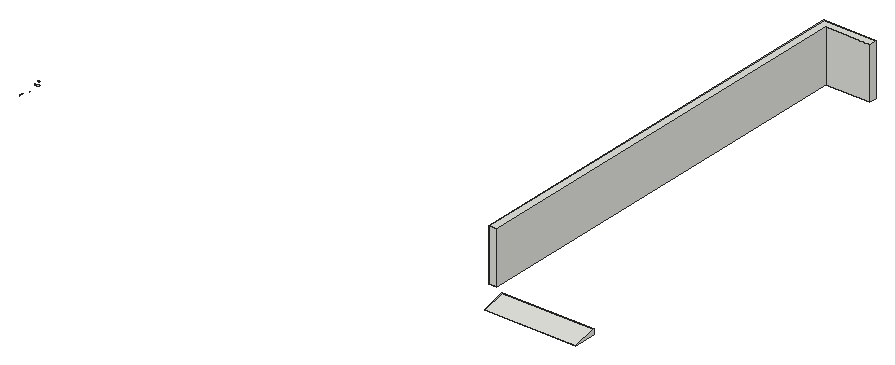
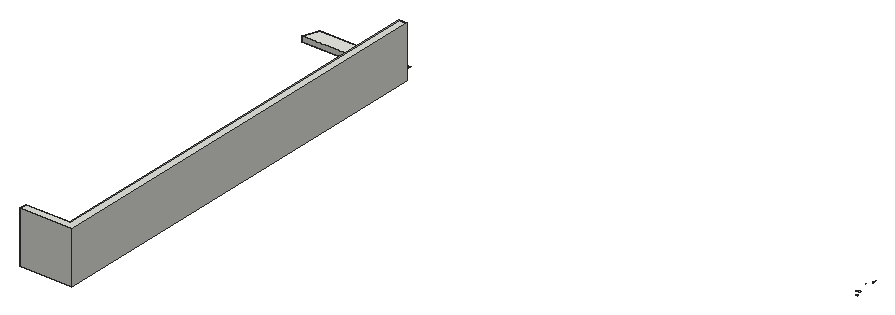
# SketchUp Ruby script. Lengths in inches.
U = 1.inch
M = Sketchup.active_model
def pt(a) = Geom::Point3d.new(a.map { |v| v * U })
def face(e, loops, mat)
  f = e.add_face(loops[0].map { |a| pt(a) })
  loops[1..].each { |l| e.add_face(l.map { |a| pt(a) }).erase! }
  f.material = f.back_material = mat if mat
  f
end
# faces: each face lists its corners as indices into pts; further lists are holes
def faces(e, pts, list, mat = nil) = list.each { |f| face(e, (f[0].is_a?(Array) ? f : [f]).map { |l| l.map { |i| pts[i] } }, mat) }
# xy, xz, yz: faces in a plane at the given z, y or x. An outline is a flat list of corners, or four numbers for a rectangle; further outlines are holes
def ring(l) = l.size == 4 ? [[l[0], l[1]], [l[2], l[1]], [l[2], l[3]], [l[0], l[3]]] : l.each_slice(2).to_a
def flat(e, list, mat, &to3) = list.each { |f| face(e, (f[0].is_a?(Array) ? f : [f]).map { |l| ring(l).map { |u, v| to3.(u, v) } }, mat) }
def xy(e, z, list, mat = nil) = flat(e, list, mat) { |x, y| [x, y, z] }
def xz(e, y, list, mat = nil) = flat(e, list, mat) { |x, z| [x, y, z] }
def yz(e, x, list, mat = nil) = flat(e, list, mat) { |y, z| [x, y, z] }
def lines(e, pts, list) = list.each { |a, b| e.add_line(pt(pts[a]), pt(pts[b])) }
# prism: a flat outline (further loops are holes) pulled along v
def prism(e, loops, v, mat = nil)
  f = face(e, loops, mat); d = Geom::Vector3d.new(v.map { |x| x * U })
  f.pushpull(f.normal.samedirection?(d) ? d.length : -d.length)
end
def box(e, o, s, mat = nil) = prism(e, [[o, [o[0] + s[0], o[1], o[2]], [o[0] + s[0], o[1] + s[1], o[2]], [o[0], o[1] + s[1], o[2]]]], [0, 0, s[2]], mat)
def at(x, y, z, deg = 0) = Geom::Transformation.translation(pt([x, y, z])) * Geom::Transformation.rotation(ORIGIN, Z_AXIS, deg.degrees)
def axes(o, x, y, z) = Geom::Transformation.new([*x, 0, *y, 0, *z, 0, *pt(o).to_a, 1])
def part(name) = M.definitions.add(name)
# library, detail: a bought-in or finely detailed component or shape, given as its bounding box
def library(name, o, s) = part(name).tap { |d| box(d.entities, o, s) }
def detail(e, o, s) = box(e.add_group.entities, o, s)
def put(e, d, t, mat = nil) = e.add_instance(d, t).tap { |i| i.material = mat if mat }
def group(e, t, mat = nil) = e.add_group.tap { |g| g.transformation = t; g.material = mat if mat }.entities
root = M.entities
prism(root,[[[600.961,339.2731,0],[600.961,313.8509,0],[600.961,339.2731,6]]],[105.6875,0,0])
xy(root,0,[[26.9831,360.1386,26.9873,360.1387,26.9915,360.1392,26.9957,360.14,26.9998,360.141,27.0039,360.1424,27.0078,360.144,27.0095,360.1449,27.0112,360.1459,27.0128,360.147,27.0143,360.1482,27.0158,360.1495,27.0172,360.1509,27.0196,360.1539,27.0207,360.1556,27.0225,360.159,27.0234,360.1614,27.0242,360.1639,27.0248,360.1663,27.0252,360.1689,27.0255,360.1714,27.0256,360.174,27.0254,360.1765,27.0251,360.1791,27.0247,360.1816,27.0232,360.1872,27.0214,360.1927,27.0192,360.198,27.0166,360.2032,27.0138,360.2082,26.995,360.2348,26.9851,360.2465,26.9744,360.2573,26.9648,360.2657,26.9547,360.2732,26.9533,360.2742,26.9517,360.275,26.9502,360.2757,26.9486,360.2764,26.9469,360.2769,26.9452,360.2773,26.9435,360.2776,26.9401,360.2778,26.939,360.2778,26.9379,360.2776,26.9368,360.2775,26.9357,360.2772,26.9347,360.2768,26.9336,360.2764,26.9326,360.276,26.9308,360.2748,26.9299,360.2741,26.9291,360.2734,26.9283,360.2726,26.9254,360.2691,26.9227,360.2654,26.9204,360.2615,26.9184,360.2573,26.9155,360.25,26.9132,360.2425,26.9116,360.2348,26.9099,360.2216,26.9094,360.2082,26.9095,360.2036,26.91,360.1991,26.9108,360.1946,26.9119,360.1902,26.9133,360.1859,26.915,360.1816,26.917,360.1775,26.9193,360.1734,26.9219,360.1695,26.9247,360.1658,26.9277,360.1623,26.931,360.159,26.9353,360.1553,26.9399,360.1519,26.9447,360.1488,26.9497,360.1462,26.9549,360.1439,26.9604,360.142,26.9659,360.1405,26.9716,360.1394,26.9773,360.1388],[27.1858,360.1773,27.1887,360.1773,27.1901,360.1774,27.1929,360.178,27.1943,360.1784,27.1956,360.1789,27.1969,360.1795,27.1998,360.1811,27.2026,360.1829,27.2053,360.1848,27.2078,360.187,27.2101,360.1893,27.2123,360.1918,27.2143,360.1944,27.2161,360.1972,27.2209,360.2058,27.225,360.2147,27.2284,360.2239,27.231,360.2334,27.2357,360.2578,27.2386,360.2826,27.243,360.3857,27.2429,360.3876,27.2427,360.3896,27.2424,360.3915,27.242,360.3934,27.2414,360.3952,27.2407,360.397,27.2398,360.3988,27.2389,360.4005,27.2367,360.4037,27.2354,360.4051,27.234,360.4065,27.2326,360.4078,27.231,360.409,27.2294,360.41,27.2277,360.411,27.2259,360.4118,27.2247,360.4123,27.2223,360.4129,27.221,360.4132,27.2198,360.4133,27.2172,360.4133,27.216,360.4132,27.2147,360.413,27.2135,360.4127,27.2111,360.4119,27.2099,360.4114,27.2088,360.4108,27.2077,360.4101,27.2057,360.4085,27.2039,360.4067,27.2031,360.4057,27.2024,360.4047,27.2017,360.4036,27.2012,360.4025,27.1634,360.3148,27.1588,360.3013,27.1551,360.2874,27.1523,360.2734,27.1508,360.26,27.1503,360.2466,27.1511,360.2332,27.1522,360.2248,27.154,360.2165,27.1563,360.2083,27.1593,360.2004,27.1606,360.1977,27.162,360.1951,27.1636,360.1926,27.1653,360.1902,27.1673,360.188,27.1693,360.1859,27.1716,360.1839,27.1739,360.1821,27.1764,360.1804,27.1776,360.1797,27.1789,360.1791,27.1802,360.1786,27.1816,360.1781,27.1844,360.1775],[27.1335,363.4794,27.1354,363.4795,27.1373,363.4797,27.1392,363.48,27.1411,363.4804,27.1429,363.481,27.1447,363.4817,27.1464,363.4825,27.1481,363.4834,27.1513,363.4856,27.1541,363.4882,27.1563,363.4908,27.1572,363.4923,27.1581,363.4937,27.1588,363.4953,27.16,363.4985,27.1604,363.5001,27.1608,363.5035,27.1609,363.5052,27.1608,363.5069,27.1606,363.5086,27.1595,363.5144,27.1581,363.5202,27.1563,363.5258,27.154,363.5312,27.1514,363.5366,27.1485,363.5417,27.134,363.5633,27.1182,363.5838,27.0868,363.6242,27.0646,363.6591,27.0582,363.6718,27.0525,363.6858,27.0523,363.6871,27.0524,363.6884,27.0528,363.6896,27.0533,363.6907,27.0541,363.6917,27.0551,363.6925,27.0562,363.6931,27.0574,363.6935,27.2123,363.7212,27.2434,363.7248,27.2746,363.726,27.3059,363.725,27.3164,363.7239,27.3268,363.7221,27.3371,363.7196,27.3471,363.7163,27.357,363.7124,27.3665,363.7079,27.3728,363.7043,27.3789,363.7004,27.3846,363.696,27.3901,363.6913,27.3953,363.6862,27.4,363.6807,27.4044,363.675,27.4085,363.669,27.4134,363.6615,27.4188,363.6544,27.4247,363.6477,27.431,363.6413,27.4349,363.6379,27.439,363.6347,27.4433,363.6319,27.4478,363.6293,27.4525,363.627,27.4572,363.625,27.4608,363.6239,27.4644,363.623,27.468,363.6223,27.4717,363.622,27.4754,363.6219,27.4791,363.622,27.4828,363.6225,27.4855,363.623,27.4881,363.6237,27.4906,363.6246,27.4931,363.6257,27.4955,363.6269,27.4979,363.6283,27.5001,363.6298,27.5022,363.6315,27.5041,363.6334,27.5072,363.6367,27.51,363.6401,27.5125,363.6438,27.5148,363.6477,27.5167,363.6517,27.5184,363.6559,27.5207,363.6631,27.5224,363.6704,27.5235,363.6779,27.524,363.6854,27.524,363.6935,27.5234,363.7015,27.5222,363.7095,27.5204,363.7173,27.5181,363.725,27.5152,363.7325,27.5118,363.7397,27.5078,363.7466,27.5013,363.7564,27.4942,363.7657,27.4864,363.7744,27.478,363.7826,27.469,363.7902,27.4596,363.7971,27.4497,363.8034,27.4393,363.809,27.4286,363.8138,27.149,363.9215,26.881,364.0111,26.8784,364.0117,26.877,364.0119,26.8757,364.012,26.8743,364.012,26.873,364.0119,26.8716,364.0117,26.869,364.0111,26.8677,364.0107,26.8664,364.0101,26.864,364.0089,26.8618,364.0073,26.8608,364.0064,26.8598,364.0054,26.8589,364.0044,26.8573,364.0022,26.8561,363.9998,26.8556,363.9985,26.8551,363.9973,26.8548,363.9959,26.8545,363.9946,26.8543,363.9933,26.8543,363.9892,26.8545,363.9879,26.8548,363.9865,26.8556,363.9839,26.8561,363.9827,26.8567,363.9815,26.8719,363.9503,26.9019,363.8799,26.9367,363.7958,26.9729,363.7056,27.0123,363.619,27.0333,363.5816,27.0569,363.5458,27.0776,363.5189,27.1003,363.4935,27.1025,363.4913,27.1049,363.4893,27.1074,363.4875,27.11,363.4859,27.1127,363.4844,27.1155,363.4831,27.1183,363.482,27.1213,363.481,27.1243,363.4803,27.1273,363.4798,27.1304,363.4795],[27.6414,363.8505,27.6432,363.8505,27.6451,363.8506,27.6469,363.8509,27.6487,363.8513,27.6504,363.8518,27.6522,363.8525,27.6538,363.8532,27.6555,363.8541,27.6574,363.8553,27.6592,363.8566,27.6609,363.8581,27.6625,363.8596,27.664,363.8613,27.6654,363.863,27.6678,363.8668,27.6688,363.8688,27.6696,363.8709,27.6703,363.873,27.6709,363.8752,27.6713,363.8774,27.6716,363.8796,27.675,363.9581,27.6741,363.9777,27.6716,363.9971,27.6674,364.0163,27.6644,364.0263,27.6606,364.0362,27.6562,364.0457,27.651,364.055,27.6453,364.0638,27.6406,364.0699,27.6355,364.0757,27.6301,364.081,27.6242,364.086,27.618,364.0906,27.6115,364.0947,27.6068,364.0973,27.6019,364.0995,27.5969,364.1014,27.5918,364.103,27.5866,364.1042,27.5813,364.1051,27.5759,364.1056,27.5706,364.1058,27.5571,364.1053,27.5438,364.1038,27.5306,364.1013,27.5218,364.0989,27.5132,364.0958,27.5049,364.0922,27.4968,364.0879,27.4917,364.0846,27.4869,364.081,27.4823,364.077,27.4781,364.0726,27.4742,364.068,27.4727,364.066,27.4714,364.0639,27.4702,364.0617,27.4691,364.0594,27.4682,364.057,27.4675,364.0546,27.4669,364.0522,27.4665,364.0497,27.4662,364.0472,27.4662,364.0447,27.4663,364.0404,27.4667,364.036,27.4675,364.0317,27.4685,364.0275,27.4698,364.0234,27.4713,364.0193,27.4732,364.0154,27.4843,363.9953,27.4968,363.9761,27.513,363.9548,27.5306,363.9347,27.5706,363.897,27.6275,363.8548,27.6307,363.853,27.6324,363.8523,27.6341,363.8517,27.6359,363.8512,27.6377,363.8508,27.6395,363.8506],[29.9973,370.1849,29.9984,370.185,29.9995,370.1853,30.0005,370.1857,30.0015,370.1862,30.0024,370.1869,30.0032,370.1877,30.0039,370.1885,30.0097,370.1978,30.0149,370.2075,30.0193,370.2175,30.0238,370.23,30.0274,370.2427,30.0302,370.2556,30.032,370.2685,30.0328,370.2814,30.0328,370.2944,30.0318,370.3058,30.03,370.3171,30.0273,370.3282,30.0261,370.3318,30.0246,370.3353,30.0229,370.3388,30.021,370.342,30.0188,370.3452,30.0164,370.3481,30.0131,370.3516,30.0116,370.3528,30.0099,370.3537,30.0081,370.3544,30.0062,370.3549,30.0043,370.3551,30.0023,370.3551,30.0004,370.3547,29.9986,370.3542,29.9972,370.3536,29.9958,370.3528,29.9944,370.3521,29.9932,370.3512,29.992,370.3502,29.9908,370.3491,29.9898,370.348,29.9888,370.3468,29.9879,370.3456,29.9871,370.3442,29.9864,370.3429,29.9857,370.3415,29.9828,370.3333,29.9806,370.325,29.979,370.3166,29.978,370.308,29.9773,370.2596,29.9814,370.2076,29.9817,370.2054,29.9822,370.2031,29.9828,370.2009,29.9836,370.1988,29.9856,370.1946,29.9868,370.1927,29.9882,370.1908,29.9896,370.189,29.9912,370.1873,29.992,370.1866,29.993,370.186,29.994,370.1855,29.995,370.1852,29.9961,370.185],
  [26.9652,383.6659,26.9695,383.6661,26.9738,383.6665,26.978,383.6673,26.9822,383.6683,26.9848,383.6692,26.9874,383.6702,26.9899,383.6714,26.9923,383.6728,26.9946,383.6743,26.9968,383.676,26.9989,383.6779,27.0008,383.6798,27.0026,383.6819,27.0043,383.6841,27.0058,383.6865,27.0072,383.6889,27.0083,383.6914,27.0093,383.694,27.0102,383.6966,27.0108,383.6993,27.0113,383.702,27.0115,383.7048,27.0116,383.7076,27.0101,383.7396,27.0059,383.7713,26.9991,383.8026,26.9957,383.8178,26.9933,383.8332,26.9919,383.8488,26.9915,383.8644,26.9922,383.88,26.9939,383.8955,26.9945,383.8987,26.9952,383.9019,26.9962,383.905,26.9974,383.9081,26.9988,383.911,27.0004,383.9139,27.0022,383.9166,27.0042,383.9192,27.0063,383.9217,27.0086,383.924,27.011,383.9262,27.0136,383.9282,27.0163,383.93,27.0191,383.9317,27.022,383.9331,27.025,383.9344,27.0281,383.9354,27.0313,383.9363,27.0345,383.9369,27.0418,383.9378,27.0492,383.9383,27.0565,383.9382,27.0639,383.9376,27.0712,383.9366,27.0784,383.935,27.0855,383.9329,27.0924,383.9304,27.0991,383.9274,27.1057,383.924,27.1119,383.9201,27.1643,383.8812,27.2126,383.8374,27.2555,383.7974,27.298,383.7637,27.3353,383.739,27.3378,383.7376,27.3403,383.7364,27.343,383.7354,27.3457,383.7345,27.3484,383.7339,27.3512,383.7334,27.354,383.7331,27.3568,383.733,27.358,383.733,27.3593,383.7332,27.3605,383.7334,27.3618,383.7337,27.363,383.734,27.3641,383.7345,27.3653,383.735,27.3675,383.7362,27.3695,383.7378,27.3704,383.7386,27.3712,383.7396,27.372,383.7405,27.3759,383.746,27.3793,383.7516,27.3823,383.7576,27.3849,383.7637,27.3886,383.7747,27.3916,383.786,27.3937,383.7974,27.3958,383.8173,27.3966,383.8374,27.3971,383.8508,27.3989,383.8642,27.4018,383.8773,27.4039,383.8844,27.4065,383.8914,27.4096,383.8982,27.4131,383.9048,27.417,383.9111,27.4201,383.9155,27.4235,383.9196,27.4272,383.9236,27.4311,383.9272,27.4353,383.9306,27.4396,383.9337,27.4426,383.9356,27.4457,383.9372,27.449,383.9386,27.4523,383.9397,27.4557,383.9406,27.4592,383.9413,27.4626,383.9417,27.4662,383.9418,27.4697,383.9417,27.4732,383.9413,27.4766,383.9406,27.48,383.9397,27.4834,383.9386,27.4866,383.9372,27.4897,383.9356,27.4927,383.9337,27.4971,383.9306,27.5012,383.9272,27.5051,383.9236,27.5088,383.9196,27.5122,383.9155,27.5153,383.9111,27.5192,383.9048,27.5227,383.8982,27.5258,383.8914,27.5284,383.8844,27.5306,383.8773,27.5334,383.8642,27.5352,383.8508,27.5358,383.8374,27.5361,383.8275,27.5372,383.8176,27.5389,383.8078,27.5414,383.7982,27.5445,383.7888,27.5483,383.7796,27.5527,383.7707,27.5552,383.7666,27.558,383.7626,27.561,383.7588,27.5643,383.7552,27.5678,383.7518,27.5715,383.7487,27.5755,383.7459,27.5796,383.7434,27.584,383.7411,27.5884,383.7392,27.593,383.7376,27.5977,383.7363,27.6026,383.7353,27.6075,383.7346,27.6125,383.7342,27.6175,383.7342,27.6225,383.7345,27.6275,383.7352,27.6324,383.7361,27.6372,383.7374,27.6419,383.739,27.6466,383.7409,27.6511,383.7431,27.6554,383.7456,27.664,383.7514,27.6721,383.7577,27.6799,383.7645,27.6872,383.7718,27.694,383.7796,27.7002,383.7878,27.706,383.7964,27.7082,383.7998,27.7106,383.803,27.7133,383.806,27.7162,383.8088,27.7192,383.8114,27.7225,383.8138,27.7259,383.8159,27.7294,383.8179,27.733,383.8195,27.7587,383.8288,27.7852,383.8356,27.8177,383.8408,27.8505,383.8433,27.8856,383.8432,27.9206,383.8406,27.9556,383.8381,27.9908,383.8383,28.0241,383.8413,28.0569,383.8473,28.075,383.852,28.0927,383.858,28.11,383.8651,28.1138,383.867,28.1175,383.8692,28.1211,383.8716,28.1245,383.8742,28.1277,383.877,28.1307,383.8801,28.1336,383.8833,28.1362,383.8867,28.1386,383.8903,28.1392,383.8915,28.1398,383.8928,28.1404,383.894,28.1408,383.8954,28.1411,383.8967,28.1414,383.8981,28.1416,383.9009,28.1415,383.9022,28.1414,383.9036,28.1412,383.905,28.1409,383.9063,28.1405,383.9077,28.1399,383.909,28.1394,383.9102,28.1387,383.9114,28.1379,383.9126,28.1371,383.9137,28.1362,383.9148,28.1352,383.9158,28.1316,383.9189,28.1278,383.9218,28.1239,383.9244,28.1197,383.9267,28.1154,383.9287,28.1109,383.9304,28.1064,383.9317,28.1017,383.9328,28.0784,383.9362,28.055,383.9379,28.0314,383.9378,27.9281,383.9297,27.7768,383.9181,27.7634,383.9181,27.75,383.9191,27.7367,383.9211,27.7235,383.9242,27.7107,383.9282,27.6982,383.9331,27.6962,383.934,27.6926,383.9362,27.6909,383.9375,27.6893,383.9389,27.6878,383.9404,27.6864,383.942,27.6851,383.9437,27.6839,383.9455,27.6829,383.9473,27.6819,383.9493,27.6811,383.9512,27.6805,383.9533,27.68,383.9553,27.6796,383.9574,27.6793,383.9595,27.6792,383.9617,27.6794,383.9659,27.6802,383.9701,27.6825,383.9777,27.6853,383.9852,27.6885,383.9925,27.6922,383.9995,27.6964,384.0063,27.701,384.0128,27.7061,384.019,27.7115,384.0248,27.7135,384.0266,27.7156,384.0283,27.7178,384.0299,27.7201,384.0313,27.7225,384.0326,27.725,384.0337,27.7276,384.0346,27.7302,384.0353,27.7328,384.0359,27.7355,384.0363,27.7382,384.0365,27.7409,384.0365,27.8406,384.0318,27.9623,384.0193,28.0996,383.9975,28.26,383.9736,28.3226,383.9685,28.3855,383.9677,28.4328,383.9708,28.4796,383.9781,28.4889,383.9804,28.498,383.9832,28.5069,383.9867,28.5155,383.9908,28.5238,383.9956,28.5317,384.0008,28.5393,384.0067,28.5511,384.0157,28.5635,384.0239,28.5766,384.031,28.586,384.0353,28.5957,384.0389,28.6056,384.0418,28.6158,384.044,28.6227,384.045,28.6297,384.0456,28.6368,384.0456,28.6438,384.0451,28.6507,384.0442,28.6539,384.0436,28.657,384.0427,28.66,384.0416,28.6629,384.0404,28.6658,384.0389,28.6685,384.0372,28.6711,384.0354,28.6736,384.0334,28.676,384.0312,28.6773,384.0299,28.6788,384.0287,28.6803,384.0277,28.6819,384.0267,28.6835,384.0258,28.6852,384.0251,28.687,384.0244,28.6888,384.0239,28.6906,384.0235,28.6924,384.0232,28.6943,384.0231,28.6962,384.0231,28.698,384.0232,28.6999,384.0234,28.7017,384.0237,28.7035,384.0242,28.7053,384.0248,28.723,384.0321,28.7401,384.0407,28.7565,384.0506,28.7883,384.0734,28.818,384.099,28.8818,384.1656,28.9154,384.2016,28.9519,384.2347,28.9909,384.2647,29.0323,384.2913,29.0706,384.3116,29.1106,384.3283,29.1207,384.3316,29.1309,384.3341,29.1414,384.3359,29.1519,384.3369,29.1625,384.3371,29.1731,384.3366,29.1903,384.3356,29.2075,384.3358,29.2246,384.3371,29.2359,384.3388,29.247,384.3413,29.258,384.3445,29.2686,384.3486,29.2752,384.3516,29.2815,384.3552,29.2875,384.3592,29.2933,384.3637,29.2986,384.3686,29.3004,384.3705,29.3021,384.3725,29.3036,384.3746,29.305,384.3768,29.3062,384.3791,29.3072,384.3815,29.3081,384.384,29.3088,384.3865,29.3094,384.389,29.3098,384.3916,29.3099,384.3942,29.3112,384.4117,29.3138,384.429,29.3175,384.4462,29.3224,384.463,29.3284,384.4795,29.3378,384.5004,29.3488,384.5204,29.3613,384.5396,29.3753,384.5578,29.3853,384.569,29.3961,384.5794,29.4078,384.5889,29.4201,384.5975,29.433,384.6051,29.436,384.6066,29.439,384.6079,29.4422,384.6089,29.4454,384.6098,29.4486,384.6105,29.4519,384.6109,29.4552,384.6111,29.4585,384.6111,29.4618,384.6109,29.4651,384.6105,29.4683,384.6099,29.4715,384.609,29.4746,384.608,29.4777,384.6067,29.4807,384.6053,29.4835,384.6036,29.4871,384.6016,29.4908,384.5998,29.4945,384.5982,29.4984,384.5969,29.5024,384.5959,29.5064,384.5951,29.5105,384.5946,29.5145,384.5943,29.5186,384.5944,29.5831,384.6007,29.6599,384.6179,29.7397,384.645,29.8611,384.6949,29.8641,384.6963,29.8669,384.6979,29.8696,384.6997,29.8722,384.7016,29.8747,384.7038,29.877,384.7061,29.8791,384.7085,29.8811,384.7111,29.8828,384.7138,29.8844,384.7166,29.8858,384.7196,29.8863,384.7207,29.8867,384.7219,29.8869,384.7232,29.8872,384.7244,29.8873,384.7257,29.8873,384.7282,29.8871,384.7294,29.8869,384.7307,29.8866,384.7319,29.8862,384.7331,29.8858,384.7342,29.8852,384.7354,29.8846,384.7365,29.8839,384.7375,29.8823,384.7395,29.8814,384.7403,29.8805,384.7412,29.8795,384.7419,29.8784,384.7426,29.8773,384.7432,29.7978,384.7798,29.7183,384.814,29.7173,384.8146,29.7163,384.8153,29.7155,384.8161,29.7147,384.817,29.7141,384.818,29.7136,384.8191,29.7133,384.8202,29.7131,384.8213,29.7131,384.8225,29.7132,384.8237,29.7135,384.8248,29.7139,384.8259,29.7145,384.8269,29.7152,384.8279,29.7165,384.8293,29.7178,384.8306,29.7193,384.8319,29.7209,384.833,29.7225,384.834,29.7242,384.8349,29.726,384.8357,29.7278,384.8364,29.7296,384.8369,29.7315,384.8373,29.7334,384.8376,29.7353,384.8378,29.85,384.8417,29.8868,384.8441,29.9232,384.8495,29.9444,384.8544,29.965,384.8609,29.9851,384.869,29.9964,384.8746,30.0073,384.8811,30.0176,384.8883,30.0273,384.8964,30.0294,384.8984,30.0314,384.9006,30.0332,384.9029,30.0349,384.9054,30.0364,384.9079,30.0377,384.9106,30.0388,384.9133,30.0397,384.9161,30.0404,384.919,30.0409,384.9219,30.0413,384.9248,30.0414,384.9278,30.041,384.9372,30.0399,384.9466,30.0382,384.9558,30.0377,384.9577,30.0371,384.9595,30.0363,384.9613,30.0355,384.963,30.0345,384.9647,30.0334,384.9663,30.0322,384.9678,30.0309,384.9692,30.0295,384.9706,30.028,384.9718,30.0272,384.9724,30.0263,384.973,30.0245,384.974,30.0215,384.9749,30.0205,384.9751,30.0194,384.9752,30.0173,384.9752,30.0163,384.9751,30.0143,384.9747,30.0133,384.9744,30.0105,384.9734,30.0053,384.9708,30.0028,384.9692,30.0004,384.9675,29.9982,384.9657,29.996,384.9637,29.9945,384.9622,29.9928,384.9608,29.9911,384.9596,29.9892,384.9585,29.9873,384.9575,29.9854,384.9566,29.9834,384.9558,29.9813,384.9552,29.9771,384.9544,29.975,384.9542,29.9728,384.9542,29.9675,384.9544,29.9621,384.955,29.9568,384.956,29.9516,384.9573,29.9465,384.959,29.9416,384.961,29.9323,384.9656,29.9234,384.9709,29.9149,384.9768,29.9068,384.9834,29.8897,385,29.8742,385.0183,29.868,385.0258,29.8613,385.0329,29.8542,385.0395,29.8465,385.0456,29.8385,385.0511,29.8301,385.056,29.8213,385.0604,29.8123,385.0641,29.8031,385.0671,29.6402,385.1054,29.402,385.1377,29.059,385.1643,28.5951,385.1896,28.5022,385.19,28.4096,385.1824,28.3905,385.1793,28.3717,385.1747,28.3533,385.1688,28.3354,385.1614,28.3181,385.1528,28.3014,385.1429,28.2814,385.1288,28.2625,385.1132,28.2449,385.0962,28.2287,385.0779,28.2139,385.0584,28.1657,384.9968,28.1602,384.9909,28.1542,384.9854,28.148,384.9802,28.1413,384.9755,28.1344,384.9713,28.1272,384.9675,28.1253,384.9667,28.1233,384.966,28.1213,384.9654,28.1192,384.9649,28.115,384.9645,28.1129,384.9645,28.1087,384.9649,28.1066,384.9654,28.1046,384.966,28.1026,384.9667,28.1006,384.9675,28.0987,384.9685,28.0962,384.9701,28.0938,384.9718,28.0915,384.9737,28.0893,384.9757,28.0873,384.9779,28.0854,384.9802,28.0837,384.9826,28.0821,384.9851,28.0807,384.9877,28.0795,384.9904,28.0785,384.9932,28.0764,384.9989,28.0739,385.0043,28.071,385.0096,28.0678,385.0147,28.0642,385.0195,28.0602,385.024,28.0574,385.0269,28.0543,385.0296,28.051,385.0321,28.0476,385.0343,28.044,385.0363,28.0403,385.038,28.0365,385.0394,28.0326,385.0406,28.0277,385.0417,28.0227,385.0424,28.0177,385.0428,28.0126,385.0428,28.0076,385.0424,28.0026,385.0417,27.9977,385.0406,27.9877,385.0376,27.9778,385.0339,27.9684,385.0294,27.9592,385.0242,27.937,385.0092,27.9159,384.9926,27.9143,384.9911,27.9128,384.9896,27.9115,384.9879,27.9102,384.9861,27.9091,384.9843,27.908,384.9823,27.9072,384.9804,27.9064,384.9783,27.9058,384.9762,27.9054,384.9741,27.9051,384.9719,27.905,384.9698,27.905,384.9676,27.9051,384.9652,27.9055,384.9628,27.906,384.9604,27.9066,384.9581,27.9075,384.9558,27.9085,384.9536,27.9096,384.9514,27.9109,384.9494,27.9123,384.9474,27.9139,384.9456,27.9156,384.9438,27.9174,384.9422,27.9398,384.9246,27.9633,384.9086,28.0025,384.8813,28.0041,384.88,28.0055,384.8787,28.0068,384.8773,28.0081,384.8757,28.0092,384.8742,28.0102,384.8725,28.0111,384.8708,28.0119,384.869,28.0126,384.8671,28.0132,384.8653,28.0137,384.8627,28.0138,384.8614,28.0137,384.86,28.0134,384.8587,28.0129,384.8575,28.0123,384.8563,28.0116,384.8552,28.0107,384.8542,28.0097,384.8533,28.0085,384.8526,28.0073,384.852,28.006,384.8516,27.9958,384.8495,27.9853,384.8482,27.9749,384.8477,27.966,384.8479,27.9572,384.8487,27.9485,384.8503,27.94,384.8524,27.9275,384.8565,27.9154,384.8615,27.9037,384.8674,27.8924,384.874,27.8817,384.8814,27.8715,384.8896,27.8652,384.8956,27.8592,384.9021,27.8538,384.9089,27.849,384.9162,27.8443,384.9232,27.8391,384.9299,27.8335,384.9362,27.8274,384.9421,27.821,384.9475,27.8142,384.9525,27.807,384.957,27.7996,384.961,27.7919,384.9645,27.7839,384.9674,27.7636,384.9733,27.7428,384.9777,27.7218,384.9806,27.7007,384.982,27.6795,384.9818,27.6456,384.9793,27.612,384.9744,27.5787,384.9674,27.546,384.9581,27.4701,384.9305,27.3966,384.897,27.3713,384.8853,27.3453,384.8755,27.3187,384.8675,27.2916,384.8615,27.1232,384.8373,26.9163,384.8245,26.6832,384.8251,26.3116,384.8294,26.2919,384.8286,26.2723,384.8265,26.253,384.823,26.2338,384.8182,26.2151,384.812,26.1968,384.8047,26.1791,384.7961,26.177,384.7949,26.175,384.7936,26.1731,384.7921,26.1713,384.7905,26.1696,384.7889,26.168,384.7871,26.1666,384.7852,26.1652,384.7832,26.164,384.7811,26.1629,384.779,26.162,384.7768,26.1612,384.7745,26.1606,384.7722,26.1601,384.7698,26.1598,384.7675,26.1596,384.7627,26.1598,384.7603,26.1601,384.7579,26.1606,384.7556,26.1612,384.7533,26.1619,384.751,26.1628,384.7488,26.1639,384.7466,26.1651,384.7446,26.1664,384.7426,26.1679,384.7407,26.1694,384.7389,26.1711,384.7372,26.1729,384.7356,26.2207,384.6987,26.2709,384.6651,26.3231,384.6349,26.3607,384.6132,26.3967,384.589,26.4694,384.5305,26.531,384.4689,26.5452,384.4518,26.5579,384.4335,26.5692,384.4143,26.5849,384.3824,26.5983,384.3493,26.5991,384.3467,26.5998,384.344,26.6003,384.3412,26.6006,384.3384,26.6007,384.3356,26.6006,384.3328,26.6004,384.33,26.5999,384.3273,26.5993,384.3246,26.5984,384.3219,26.5974,384.3193,26.5962,384.3167,26.5949,384.3143,26.5917,384.3097,26.5898,384.3076,26.5878,384.3056,26.5857,384.3038,26.5835,384.302,26.5812,384.3005,26.5787,384.2991,26.5762,384.2979,26.5736,384.2969,26.571,384.296,26.5682,384.2953,26.5655,384.2948,26.5299,384.2911,26.4942,384.2898,26.4677,384.2908,26.4413,384.2937,26.4152,384.2986,26.4101,384.3,26.4051,384.3017,26.4002,384.3037,26.3954,384.3061,26.3909,384.3089,26.3866,384.3119,26.3824,384.3153,26.3786,384.3189,26.375,384.3228,26.3716,384.327,26.368,384.3322,26.3648,384.3376,26.3619,384.3433,26.3595,384.3491,26.3574,384.3551,26.3558,384.3612,26.3545,384.3674,26.3537,384.3737,26.3534,384.38,26.354,384.4264,26.3583,384.4726,26.3588,384.4771,26.3589,384.4817,26.3587,384.4863,26.3582,384.4908,26.3574,384.4953,26.3564,384.4998,26.355,384.5041,26.3533,384.5084,26.3513,384.5125,26.3491,384.5165,26.3466,384.5204,26.3438,384.524,26.3408,384.5275,26.3376,384.5307,26.3342,384.5338,26.3305,384.5365,26.1583,384.6499,25.9764,384.7485,25.9614,384.7551,25.946,384.7606,25.9302,384.7649,25.9142,384.7682,25.898,384.7703,25.8817,384.7712,25.8654,384.771,25.819,384.7674,25.8171,384.767,25.8153,384.7665,25.8136,384.7656,25.812,384.7646,25.8105,384.7634,25.8093,384.762,25.8082,384.7604,25.8073,384.7587,25.807,384.7576,25.8067,384.7564,25.8067,384.7552,25.8068,384.754,25.807,384.7529,25.8074,384.7518,25.808,384.7507,25.8087,384.7498,25.8095,384.7489,25.8104,384.7482,25.8114,384.7476,25.8484,384.7308,25.8538,384.7283,25.8591,384.7256,25.8642,384.7225,25.869,384.7191,25.8737,384.7153,25.878,384.7113,25.8814,384.7078,25.8845,384.7041,25.8873,384.7002,25.8899,384.6961,25.8922,384.6918,25.8942,384.6874,25.896,384.6829,25.8974,384.6783,25.8985,384.6737,25.8993,384.669,25.8997,384.6642,25.8999,384.6594,25.8997,384.6547,25.8992,384.6499,25.8982,384.6442,25.8969,384.6386,25.8951,384.633,25.8929,384.6276,25.8904,384.6224,25.8876,384.6174,25.8712,384.5885,25.8571,384.5585,25.8454,384.5274,25.8361,384.4956,25.8291,384.4624,25.8244,384.4289,25.8223,384.3951,25.8225,384.3612,25.8243,384.3398,25.8276,384.3186,25.8326,384.2978,25.8391,384.2773,25.8472,384.2575,25.8491,384.2536,25.8512,384.2499,25.8536,384.2464,25.8562,384.243,25.8591,384.2398,25.8621,384.2368,25.8654,384.2341,25.8688,384.2315,25.8724,384.2292,25.8761,384.2271,25.88,384.2253,25.884,384.2238,25.888,384.2225,25.8922,384.2215,25.8964,384.2208,25.9006,384.2203,25.9049,384.2202,25.9177,384.2196,25.9305,384.218,25.943,384.2153,25.9515,384.2127,25.9597,384.2095,25.9677,384.2056,25.9753,384.201,25.9794,384.1981,25.9834,384.1949,25.9871,384.1915,25.9906,384.1878,25.9939,384.1839,25.9969,384.1798,25.9985,384.1773,25.9999,384.1747,26.0011,384.1721,26.0021,384.1693,26.003,384.1665,26.0037,384.1637,26.0042,384.1608,26.0045,384.1579,26.0046,384.1549,26.0044,384.1513,26.0041,384.1476,26.0034,384.144,26.0026,384.1405,26.0015,384.137,26.0001,384.1336,25.9986,384.1303,25.9968,384.1271,25.9948,384.1241,25.9926,384.1212,25.9902,384.1184,25.9876,384.1158,25.9848,384.1134,25.9819,384.1112,25.9789,384.1092,25.9757,384.1074,25.9724,384.1059,25.969,384.1045,25.9655,384.1034,25.962,384.1026,25.9437,384.0995,25.9252,384.0976,25.9066,384.0971,25.8881,384.0979,25.8697,384.1,25.8514,384.1034,25.8262,384.11,25.8015,384.1181,25.7773,384.1279,25.7539,384.1393,25.7313,384.1522,25.7239,384.1571,25.7168,384.1625,25.7102,384.1684,25.704,384.1747,25.6982,384.1814,25.6929,384.1886,25.6881,384.1961,25.6839,384.2038,25.6802,384.2119,25.677,384.2202,25.6745,384.2287,25.672,384.237,25.669,384.245,25.6654,384.2528,25.6613,384.2603,25.6567,384.2675,25.6516,384.2744,25.646,384.2809,25.6387,384.2883,25.6309,384.2951,25.6225,384.3013,25.6138,384.3069,25.6047,384.3119,25.5952,384.3162,25.5764,384.3231,25.5571,384.3286,25.5374,384.3326,25.5174,384.3352,25.4067,384.3385,25.3157,384.3319,25.2772,384.326,25.2391,384.3174,25.211,384.3088,25.1838,384.2981,25.1823,384.2973,25.1809,384.2965,25.1795,384.2956,25.1782,384.2946,25.177,384.2936,25.1758,384.2924,25.1747,384.2912,25.1737,384.2898,25.1728,384.2885,25.172,384.287,25.1713,384.2856,25.1707,384.284,25.1702,384.2825,25.1696,384.2793,25.1694,384.2776,25.1694,384.276,25.1693,384.2739,25.1691,384.2717,25.1687,384.2696,25.1682,384.2676,25.1675,384.2655,25.1668,384.2635,25.1658,384.2616,25.1648,384.2598,25.1636,384.258,25.1623,384.2563,25.1609,384.2547,25.1565,384.2504,25.1519,384.2464,25.147,384.2428,25.1419,384.2395,25.1365,384.2366,25.1278,384.2326,25.1188,384.2292,25.1097,384.2264,25.1003,384.2243,25.079,384.2212,25.0575,384.2202,25.0461,384.2206,25.0349,384.2219,25.0237,384.2241,25.0127,384.2272,25.0094,384.2283,25.0062,384.2297,25.0031,384.2313,25.0001,384.2331,24.9973,384.2351,24.9946,384.2373,24.992,384.2397,24.9896,384.2422,24.9874,384.2449,24.9853,384.2478,24.9835,384.2507,24.9818,384.2538,24.9803,384.2571,24.9791,384.2604,24.9781,384.2637,24.9773,384.2672,24.9767,384.2706,24.9764,384.2741,24.9763,384.2777,24.9764,384.2812,24.9776,384.2927,24.9797,384.3041,24.9826,384.3153,24.9863,384.3262,24.9954,384.3524,25.0025,384.3793,25.0027,384.3803,25.0029,384.3823,25.0029,384.3833,25.0028,384.3844,25.0027,384.3854,25.0025,384.3864,25.0022,384.3874,25.0018,384.3883,25.0014,384.3893,25.001,384.3902,25.0004,384.3911,24.9999,384.3919,24.9985,384.3935,24.9978,384.3942,24.997,384.3949,24.9962,384.3955,24.9944,384.3965,24.9935,384.3969,24.9925,384.3973,24.99,384.3981,24.9874,384.3987,24.9847,384.3991,24.9821,384.3994,24.9794,384.3994,24.9767,384.3993,24.9741,384.399,24.9715,384.3985,24.9689,384.3978,24.9664,384.3969,24.9639,384.3959,24.891,384.3594,24.8112,384.3118,24.8088,384.3101,24.8064,384.3082,24.8042,384.3061,24.8022,384.3039,24.8003,384.3015,24.7986,384.299,24.7971,384.2964,24.7957,384.2937,24.7946,384.2909,24.7936,384.2881,24.7929,384.2852,24.7923,384.2822,24.792,384.2792,24.7918,384.2754,24.7919,384.2717,24.7923,384.2679,24.7929,384.2642,24.7938,384.2606,24.7949,384.257,24.7963,384.2535,24.798,384.2501,24.7999,384.2469,24.802,384.2438,24.8043,384.2408,24.8752,384.1626,24.8988,384.14,24.9242,384.1194,24.9355,384.1115,24.9473,384.1044,24.9596,384.0981,24.9722,384.0926,24.9798,384.0899,24.9876,384.0878,24.9956,384.0864,25.0036,384.0855,25.0117,384.0853,25.0138,384.0854,25.0159,384.0856,25.018,384.086,25.02,384.0865,25.022,384.0872,25.024,384.088,25.0259,384.0889,25.0277,384.0899,25.0294,384.0911,25.0311,384.0924,25.0327,384.0938,25.0341,384.0953,25.0355,384.0969,25.0368,384.0986,25.0389,384.1015,25.0412,384.1041,25.0437,384.1067,25.0464,384.109,25.0492,384.1111,25.0522,384.1131,25.0553,384.1148,25.0585,384.1163,25.0618,384.1176,25.0652,384.1186,25.0834,384.1227,25.1018,384.1257,25.1203,384.1274,25.1548,384.128,25.1892,384.1256,25.2263,384.1202,25.263,384.1123,25.3414,384.0974,25.3558,384.096,25.3703,384.0958,25.3848,384.0965,25.3991,384.0984,25.4039,384.0994,25.4086,384.1006,25.4133,384.1022,25.4178,384.1041,25.4221,384.1062,25.4263,384.1087,25.4304,384.1114,25.4343,384.1144,25.4361,384.1161,25.4379,384.1179,25.4396,384.1198,25.4411,384.1218,25.4424,384.1239,25.4437,384.1261,25.4447,384.1284,25.4456,384.1307,25.4464,384.1331,25.447,384.1355,25.4474,384.138,25.4477,384.1405,25.4478,384.143,25.4479,384.1481,25.4484,384.1531,25.4492,384.1581,25.4504,384.163,25.4519,384.1678,25.4536,384.1725,25.4562,384.178,25.4592,384.1833,25.4625,384.1883,25.4663,384.1931,25.4704,384.1975,25.4749,384.2016,25.4796,384.2054,25.4847,384.2088,25.49,384.2118,25.4955,384.2143,25.5002,384.2161,25.505,384.2176,25.5099,384.2187,25.5149,384.2195,25.5199,384.22,25.5249,384.2202,25.5274,384.2201,25.5298,384.2199,25.5322,384.2195,25.5346,384.2189,25.537,384.2182,25.5393,384.2173,25.5415,384.2163,25.5437,384.2151,25.5458,384.2138,25.5478,384.2124,25.5497,384.2108,25.5515,384.2091,25.5531,384.2073,25.5565,384.2031,25.5596,384.1986,25.5623,384.194,25.5647,384.1891,25.5667,384.1841,25.5683,384.1789,25.5696,384.1736,25.5717,384.1601,25.5727,384.1465,25.5728,384.1328,25.5717,384.1192,25.5664,384.0831,25.5587,384.0475,25.536,383.9417,25.5357,383.9396,25.5356,383.9375,25.5356,383.9354,25.5357,383.9333,25.536,383.9312,25.5364,383.9291,25.5369,383.9271,25.5376,383.9251,25.5384,383.9231,25.5394,383.9212,25.5404,383.9194,25.5416,383.9177,25.5429,383.916,25.5444,383.9144,25.5459,383.913,25.5475,383.9116,25.5492,383.9104,25.5517,383.9088,25.5544,383.9073,25.5571,383.9061,25.5599,383.9051,25.5628,383.9042,25.5657,383.9036,25.5687,383.9032,25.5717,383.903,25.5747,383.903,25.5777,383.9032,25.5806,383.9036,25.5836,383.9042,25.5864,383.9051,25.7057,383.9472,25.806,383.9791,25.8193,383.982,25.8328,383.9839,25.8464,383.9847,25.8601,383.9844,25.8736,383.9831,25.8818,383.9817,25.8897,383.9798,25.8975,383.9772,25.9051,383.974,25.9125,383.9703,25.9195,383.9661,25.9262,383.9613,25.9398,383.9501,25.9526,383.938,25.9645,383.9249,25.9754,383.9111,25.9864,383.8971,25.9985,383.884,26.0114,383.8718,26.0253,383.8606,26.0399,383.8504,26.0553,383.8414,26.0713,383.8335,26.0921,383.8251,26.1135,383.818,26.1353,383.8125,26.1574,383.8084,26.1797,383.8058,26.2022,383.8048,26.2163,383.8052,26.2303,383.8064,26.2442,383.8086,26.258,383.8117,26.2715,383.8157,26.2847,383.8207,26.2975,383.8265,26.3099,383.8331,26.315,383.8363,26.3198,383.8398,26.3243,383.8436,26.3286,383.8477,26.3326,383.8522,26.3363,383.8568,26.3396,383.8618,26.3426,383.8669,26.3452,383.8723,26.3474,383.8778,26.3493,383.8835,26.3507,383.8893,26.3517,383.8951,26.3524,383.901,26.3526,383.907,26.353,383.9171,26.3542,383.9272,26.3563,383.9372,26.3591,383.9469,26.3619,383.9543,26.3652,383.9614,26.369,383.9682,26.3733,383.9748,26.3781,383.981,26.3822,383.9856,26.3865,383.9899,26.3911,383.9939,26.396,383.9976,26.4011,384.0009,26.4064,384.004,26.4108,384.0061,26.4154,384.0079,26.4201,384.0095,26.4249,384.0107,26.4297,384.0116,26.4346,384.0121,26.4396,384.0123,26.4842,384.0157,26.5505,384.0262,26.6241,384.041,26.6949,384.0583,26.7866,384.0793,26.79,384.0798,26.7935,384.0801,26.797,384.0802,26.8004,384.08,26.8039,384.0795,26.8073,384.0789,26.8107,384.0779,26.814,384.0768,26.8172,384.0754,26.8203,384.0738,26.8232,384.072,26.8247,384.071,26.8261,384.0698,26.8274,384.0686,26.8286,384.0673,26.8297,384.066,26.8308,384.0645,26.8317,384.063,26.8333,384.0598,26.8339,384.0582,26.8344,384.0565,26.8348,384.0547,26.8351,384.053,26.8353,384.0494,26.8352,384.0476,26.835,384.0459,26.8347,384.0441,26.8264,384.0112,26.8155,383.979,26.8109,383.9657,26.8073,383.9521,26.8047,383.9382,26.8031,383.9243,26.8023,383.9038,26.8029,383.8834,26.8051,383.863,26.8087,383.8432,26.8138,383.8238,26.8203,383.8047,26.8255,383.7925,26.8318,383.7808,26.839,383.7696,26.8471,383.759,26.8845,383.7179,26.9254,383.6803,26.9288,383.6777,26.9324,383.6753,26.9362,383.6731,26.94,383.6713,26.944,383.6696,26.9481,383.6683,26.9523,383.6673,26.9566,383.6665,26.9609,383.6661],[24.4989,384.1745,24.5,384.1746,24.5011,384.1749,24.5021,384.1753,24.5031,384.1758,24.504,384.1765,24.5048,384.1773,24.5055,384.1781,24.5113,384.1874,24.5165,384.1971,24.5209,384.2071,24.5254,384.2196,24.529,384.2323,24.5318,384.2452,24.5336,384.2581,24.5344,384.271,24.5344,384.284,24.5334,384.2954,24.5316,384.3067,24.5289,384.3178,24.5277,384.3214,24.5262,384.3249,24.5245,384.3284,24.5226,384.3316,24.5204,384.3348,24.518,384.3377,24.5147,384.3412,24.5132,384.3424,24.5115,384.3433,24.5097,384.344,24.5078,384.3445,24.5059,384.3447,24.5039,384.3447,24.502,384.3443,24.5002,384.3438,24.4988,384.3432,24.4974,384.3424,24.496,384.3417,24.4948,384.3408,24.4936,384.3398,24.4924,384.3387,24.4914,384.3376,24.4904,384.3364,24.4895,384.3352,24.4887,384.3338,24.488,384.3325,24.4873,384.3311,24.4844,384.3229,24.4822,384.3146,24.4806,384.3062,24.4796,384.2976,24.4789,384.2492,24.483,384.1972,24.4833,384.195,24.4838,384.1927,24.4844,384.1905,24.4852,384.1884,24.4872,384.1842,24.4884,384.1823,24.4898,384.1804,24.4912,384.1786,24.4928,384.1769,24.4936,384.1762,24.4946,384.1756,24.4956,384.1751,24.4966,384.1748,24.4977,384.1746],[27.4924,384.2898,27.5012,384.2901,27.51,384.2911,27.5187,384.2927,27.5272,384.2949,27.5355,384.2977,27.5435,384.3011,27.5512,384.3051,27.5586,384.3097,27.5656,384.3148,27.5722,384.3205,27.5772,384.3254,27.5818,384.3306,27.5861,384.3362,27.5901,384.342,27.5936,384.3481,27.5967,384.3544,27.5993,384.3607,27.6015,384.3672,27.6032,384.3738,27.6044,384.3805,27.6051,384.3874,27.6054,384.3942,27.6035,384.4342,27.6012,384.4512,27.5976,384.4679,27.594,384.4802,27.5893,384.492,27.5877,384.4946,27.5866,384.4957,27.5854,384.4966,27.5842,384.4974,27.5828,384.498,27.5813,384.4984,27.5798,384.4986,27.5775,384.4985,27.5759,384.4984,27.5744,384.4981,27.5728,384.4977,27.5713,384.4973,27.5699,384.4967,27.5684,384.496,27.567,384.4952,27.5657,384.4944,27.5645,384.4934,27.5351,384.4679,27.5013,384.4342,27.4662,384.3942,27.4231,384.3377,27.4219,384.3359,27.4208,384.3339,27.4198,384.3319,27.419,384.3298,27.4183,384.3277,27.4178,384.3255,27.4174,384.3233,27.4171,384.3211,27.417,384.3188,27.417,384.3166,27.4172,384.3143,27.4175,384.3121,27.418,384.3099,27.4184,384.3086,27.4189,384.3072,27.4194,384.3059,27.4208,384.3035,27.4216,384.3023,27.4225,384.3012,27.4235,384.3001,27.4245,384.2991,27.4256,384.2982,27.4267,384.2974,27.4279,384.2966,27.4292,384.2959,27.4305,384.2953,27.4318,384.2948,27.4331,384.2944,27.4359,384.2938,27.4641,384.2908],[25.0441,390.9096,25.2316,390.9116,25.2907,390.9172,25.3492,390.9269,25.3516,390.9275,25.354,390.9282,25.3563,390.9291,25.3585,390.9302,25.3607,390.9314,25.3628,390.9327,25.3648,390.9342,25.3666,390.9358,25.3684,390.9376,25.37,390.9394,25.3715,390.9414,25.3729,390.9435,25.3741,390.9456,25.3752,390.9478,25.3761,390.9501,25.3768,390.9525,25.3774,390.9549,25.3778,390.9573,25.3781,390.9598,25.3782,390.9623,25.3781,390.9646,25.3778,390.967,25.3775,390.9693,25.3769,390.9716,25.3762,390.9739,25.3754,390.9761,25.3744,390.9783,25.3733,390.9804,25.372,390.9824,25.3707,390.9843,25.3675,390.9879,25.3658,390.9895,25.364,390.991,25.362,390.9924,25.36,390.9936,25.3579,390.9947,25.3219,391.0104,25.2846,391.0227,25.2321,391.0353,25.1789,391.044,25.0476,391.0551,24.6903,391.0722,24.3797,391.0915,24.0852,391.1147,23.7774,391.1442,23.6142,391.1614,23.4406,391.1806,23.2814,391.1987,23.1684,391.2124,23.0816,391.2194,23.0451,391.2194,23.0086,391.2166,22.9823,391.2123,22.9565,391.2057,22.9552,391.2053,22.9539,391.2047,22.9527,391.2041,22.9516,391.2034,22.9504,391.2027,22.9474,391.2,22.9465,391.1989,22.9457,391.1978,22.945,391.1967,22.9443,391.1955,22.9438,391.1943,22.9433,391.193,22.9429,391.1917,22.9423,391.1891,22.9422,391.1877,22.9422,391.1864,22.9423,391.1828,22.9426,391.1792,22.9432,391.1757,22.9441,391.1722,22.9452,391.1687,22.9465,391.1654,22.948,391.1621,22.9497,391.159,22.9517,391.1559,22.9538,391.1531,22.9561,391.1503,22.9587,391.1478,22.9613,391.1454,22.9642,391.1432,22.9671,391.1411,22.9703,391.1393,22.9735,391.1377,22.9768,391.1364,22.9802,391.1352,22.9837,391.1343,22.9872,391.1336,23.5287,391.0515,24.1278,390.9774,24.7523,390.9248]])
g1 = group(root,at(580.5,339.27,6))
prism(g1,[[[0,6.25,0],[0,490.5,0],[60,490.5,0],[60,481.5,0],[9,481.5,0],[9,6.25,0]]],[0,0,60])
